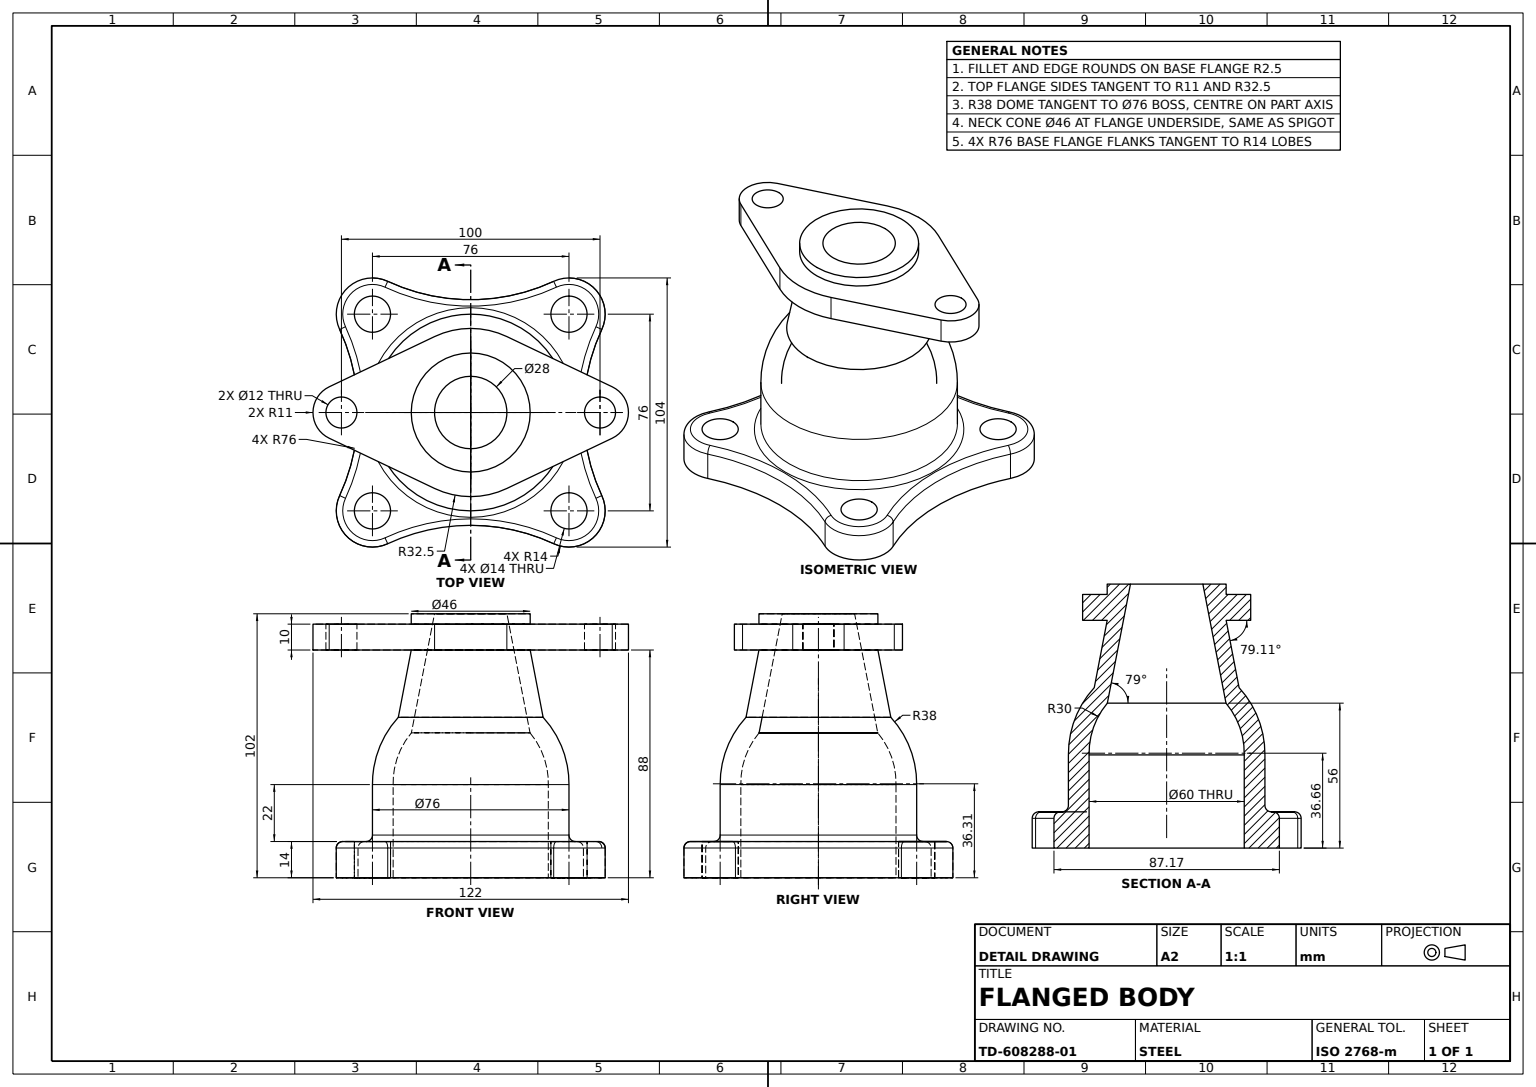
solid
v1 (0,0,-30)
v2 (0,36,-30)
e1 v1 v2 LINE
v3 (0,0,30)
e2 v3 v1 CIRCLE(AX(P(0,0,0),D(0,1,0),D(0,0,1)),30)
v4 (0,36,30)
e3 v3 v4 LINE
e4 v4 v2 CIRCLE(AX(P(0,36,0),D(0,1,0),D(0,0,1)),30)
face CYL(AX(P(0,0,0),D(0,1,0),D(0,0,1)),30) rev [-e1 -e2 e3 e4]
v5 (-38,0,45)
v6 (-38,14,45)
e5 v5 v6 LINE
v7 (-38,14,31)
e6 v6 v7 CIRCLE(AX(P(-38,14,38),D(0,1,0),D(0,0,1)),7)
v8 (-38,0,31)
e7 v8 v7 LINE
e8 v5 v8 CIRCLE(AX(P(-38,0,38),D(0,1,0),D(0,0,1)),7)
face CYL(AX(P(-38,0,38),D(0,1,0),D(0,0,1)),7) rev [e5 e6 -e7 -e8]
v9 (38,0,31)
v10 (38,14,31)
e9 v9 v10 LINE
v11 (38,0,45)
e10 v11 v9 CIRCLE(AX(P(38,0,38),D(0,1,0),D(0,0,1)),7)
v12 (38,14,45)
e11 v11 v12 LINE
e12 v12 v10 CIRCLE(AX(P(38,14,38),D(0,1,0),D(0,0,1)),7)
face CYL(AX(P(38,0,38),D(0,1,0),D(0,0,1)),7) rev [-e9 -e10 e11 e12]
v13 (0,11.5,43.584312)
v14 (0,14,41.084312)
e13 v13 v14 CIRCLE(AX(P(0,11.5,41.084312),D(-1,0,0),D(0,0,1)),2.5)
v15 (32.088889,11.5,50.690893)
e14 v15 v13 CIRCLE(AX(P(0,11.5,119.584312),D(0,1,0),D(0,0,-1)),76)
v16 (33.144444,14,48.424662)
e15 v16 v15 CIRCLE(AX(P(33.144444,11.5,48.424662),D(0.906492358,0,0.422222222),D(0.422222222,0,-0.906492358)),2.5)
e16 v14 v16 CIRCLE(AX(P(0,14,119.584312),D(0,-1,0),D(0,0,-1)),78.5)
face TORUS(AX(P(0,11.5,119.584312),D(0,-1,0),D(0,0,-1)),78.5,2.5) [-e13 -e14 -e15 -e16]
v17 (0,102,-14)
v18 (0,56,-22.941494)
e17 v17 v18 LINE
v19 (0,56,22.941494)
e18 v19 v18 CIRCLE(AX(P(0,56,0),D(0,1,0),D(0,0,1)),22.941494)
v20 (0,102,14)
e19 v20 v19 LINE
e20 v20 v17 CIRCLE(AX(P(0,102,0),D(0,1,0),D(0,0,1)),14)
face CONE(AX(P(0,56,0),D(0,-1,0),D(0,0,-1)),22.94149422,0.191986218) rev [e17 -e18 -e19 e20]
v21 (-48.424662,14,33.144444)
v22 (-33.144444,14,48.424662)
e21 v21 v22 CIRCLE(AX(P(-38,14,38),D(0,1,0),D(0,0,-1)),11.5)
v23 (-50.690893,11.5,32.088889)
e22 v21 v23 CIRCLE(AX(P(-48.424662,11.5,33.144444),D(-0.422222222,0,0.906492358),D(0.906492358,0,0.422222222)),2.5)
v24 (-32.088889,11.5,50.690893)
e23 v24 v23 CIRCLE(AX(P(-38,11.5,38),D(0,-1,0),D(0,0,-1)),14)
e24 v22 v24 CIRCLE(AX(P(-33.144444,11.5,48.424662),D(0.906492358,0,-0.422222222),D(-0.422222222,0,-0.906492358)),2.5)
face TORUS(AX(P(-38,11.5,38),D(0,-1,0),D(0,0,-1)),11.5,2.5) [-e21 e22 -e23 -e24]
v25 (54.73,98,-9.931118)
v26 (54.73,88,-9.931118)
e25 v25 v26 LINE
v27 (13.975,88,-29.341939)
e26 v26 v27 LINE
v28 (13.975,98,-29.341939)
e27 v28 v27 LINE
e28 v25 v28 LINE
face PLANE(AX(P(13.975,98,-29.341939),D(-0.43,0,0.902828887),D(0.902828887,0,0.43))) rev [e25 e26 -e27 -e28]
v29 (-38,11.5,-52)
v30 (-32.088889,11.5,-50.690893)
e29 v29 v30 CIRCLE(AX(P(-38,11.5,-38),D(0,-1,0),D(0,0,-1)),14)
v31 (-32.088889,0,-50.690893)
e30 v30 v31 LINE
v32 (-38,0,-52)
e31 v31 v32 CIRCLE(AX(P(-38,0,-38),D(0,1,0),D(0,0,1)),14)
e32 v29 v32 LINE
face CYL(AX(P(-38,14,-38),D(0,-1,0),D(0,0,-1)),14) [e29 e30 e31 -e32]
v33 (0,36,38)
v34 (0,16.5,38)
e33 v33 v34 LINE
v35 (0,16.5,-38)
e34 v34 v35 CIRCLE(AX(P(0,16.5,0),D(0,1,0),D(0,0,-1)),38)
v36 (0,36,-38)
e35 v36 v35 LINE
e36 v33 v36 CIRCLE(AX(P(0,36,0),D(0,1,0),D(0,0,1)),38)
face CYL(AX(P(0,36,0),D(0,-1,0),D(0,0,-1)),38) [e33 e34 -e35 -e36]
e37 v9 v11 CIRCLE(AX(P(38,0,38),D(0,1,0),D(0,0,1)),7)
e38 v10 v12 CIRCLE(AX(P(38,14,38),D(0,1,0),D(0,0,1)),7)
face CYL(AX(P(38,0,38),D(0,1,0),D(0,0,1)),7) rev [-e11 -e37 e9 e38]
e39 v17 v20 CIRCLE(AX(P(0,102,0),D(0,1,0),D(0,0,1)),14)
e40 v18 v19 CIRCLE(AX(P(0,56,0),D(0,1,0),D(0,0,1)),22.941494)
face CONE(AX(P(0,56,0),D(0,-1,0),D(0,0,-1)),22.94149422,0.191986218) rev [-e17 e39 e19 -e40]
v37 (50.690893,11.5,32.088889)
e41 v37 v15 CIRCLE(AX(P(38,11.5,38),D(0,-1,0),D(0,0,-1)),14)
v38 (48.424662,14,33.144444)
e42 v37 v38 CIRCLE(AX(P(48.424662,11.5,33.144444),D(0.422222222,0,0.906492358),D(0.906492358,0,-0.422222222)),2.5)
e43 v16 v38 CIRCLE(AX(P(38,14,38),D(0,1,0),D(0,0,-1)),11.5)
face TORUS(AX(P(38,11.5,38),D(0,-1,0),D(0,0,-1)),11.5,2.5) [e15 -e41 e42 -e43]
v39 (54.73,98,9.931118)
v40 (54.73,88,9.931118)
e44 v39 v40 LINE
v41 (13.975,98,29.341939)
e45 v41 v39 LINE
v42 (13.975,88,29.341939)
e46 v41 v42 LINE
e47 v42 v40 LINE
face PLANE(AX(P(13.975,98,29.341939),D(-0.43,0,-0.902828887),D(-0.902828887,0,0.43))) rev [-e44 -e45 e46 e47]
v43 (32.088889,0,50.690893)
e48 v15 v43 LINE
v44 (50.690893,0,32.088889)
e49 v43 v44 CIRCLE(AX(P(38,0,38),D(0,1,0),D(0,0,1)),14)
e50 v37 v44 LINE
face CYL(AX(P(38,14,38),D(0,-1,0),D(0,0,-1)),14) [e41 e48 e49 -e50]
v45 (-54.73,98,9.931118)
v46 (-13.975,98,29.341939)
e51 v45 v46 LINE
v47 (-54.73,88,9.931118)
e52 v45 v47 LINE
v48 (-13.975,88,29.341939)
e53 v47 v48 LINE
e54 v46 v48 LINE
face PLANE(AX(P(-54.73,98,9.931118),D(0.43,0,-0.902828887),D(-0.902828887,0,-0.43))) rev [-e51 e52 e53 -e54]
v49 (-50,98,-6)
v50 (-50,98,6)
e55 v49 v50 CIRCLE(AX(P(-50,98,0),D(0,1,0),D(0,0,1)),6)
e56 v50 v49 CIRCLE(AX(P(-50,98,0),D(0,1,0),D(0,0,1)),6)
v51 (-13.975,98,-29.341939)
v52 (-54.73,98,-9.931118)
e57 v51 v52 LINE
e58 v52 v45 CIRCLE(AX(P(-50,98,0),D(0,1,0),D(0,0,1)),11)
e59 v46 v41 CIRCLE(AX(P(0,98,0),D(0,1,0),D(0,0,1)),32.5)
e60 v39 v25 CIRCLE(AX(P(50,98,0),D(0,1,0),D(0,0,1)),11)
v53 (0,98,-32.5)
e61 v28 v53 CIRCLE(AX(P(0,98,0),D(0,1,0),D(0,0,1)),32.5)
e62 v53 v51 CIRCLE(AX(P(0,98,0),D(0,1,0),D(0,0,1)),32.5)
v54 (0,98,-23)
v55 (0,98,23)
e63 v54 v55 CIRCLE(AX(P(0,98,0),D(0,1,0),D(0,0,1)),23)
e64 v55 v54 CIRCLE(AX(P(0,98,0),D(0,1,0),D(0,0,1)),23)
v56 (50,98,6)
v57 (50,98,-6)
e65 v56 v57 CIRCLE(AX(P(50,98,0),D(0,1,0),D(0,0,1)),6)
e66 v57 v56 CIRCLE(AX(P(50,98,0),D(0,1,0),D(0,0,1)),6)
face PLANE(AX(P(-50,98,0),D(0,1,0),D(0,0,1))) [-e55 -e56] [e57 e58 e51 e59 e45 e60 e28 e61 e62] [-e63 -e64] [-e65 -e66]
v58 (-38,14,-49.5)
e67 v58 v29 CIRCLE(AX(P(-38,11.5,-49.5),D(-1,0,0),D(0,0,1)),2.5)
v59 (-33.144444,14,-48.424662)
e68 v59 v58 CIRCLE(AX(P(-38,14,-38),D(0,1,0),D(0,0,-1)),11.5)
e69 v30 v59 CIRCLE(AX(P(-33.144444,11.5,-48.424662),D(0.906492358,0,0.422222222),D(0.422222222,0,-0.906492358)),2.5)
face TORUS(AX(P(-38,11.5,-38),D(0,-1,0),D(0,0,-1)),11.5,2.5) [-e29 -e67 -e68 -e69]
v60 (50.690893,11.5,-32.088889)
e70 v60 v37 CIRCLE(AX(P(119.584312,11.5,0),D(0,1,0),D(0,0,-1)),76)
v61 (48.424662,14,-33.144444)
e71 v60 v61 CIRCLE(AX(P(48.424662,11.5,-33.144444),D(-0.422222222,0,0.906492358),D(0.906492358,0,0.422222222)),2.5)
e72 v38 v61 CIRCLE(AX(P(119.584312,14,0),D(0,-1,0),D(0,0,-1)),78.5)
face TORUS(AX(P(119.584312,11.5,0),D(0,-1,0),D(0,0,-1)),78.5,2.5) [-e70 e71 -e72 -e42]
v62 (0,102,-23)
v63 (0,102,23)
e73 v62 v63 CIRCLE(AX(P(0,102,0),D(0,1,0),D(0,0,1)),23)
e74 v63 v62 CIRCLE(AX(P(0,102,0),D(0,1,0),D(0,0,1)),23)
face PLANE(AX(P(0,102,0),D(0,1,0),D(0,0,1))) [-e39 -e20] [e73 e74]
v64 (38,0,-52)
v65 (32.088889,0,-50.690893)
e75 v64 v65 CIRCLE(AX(P(38,0,-38),D(0,1,0),D(0,0,1)),14)
v66 (32.088889,11.5,-50.690893)
e76 v66 v65 LINE
v67 (38,11.5,-52)
e77 v66 v67 CIRCLE(AX(P(38,11.5,-38),D(0,-1,0),D(0,0,-1)),14)
e78 v67 v64 LINE
face CYL(AX(P(38,14,-38),D(0,-1,0),D(0,0,-1)),14) [e75 -e76 e77 e78]
v68 (0,14,40.5)
e79 v68 v34 CIRCLE(AX(P(0,16.5,40.5),D(1,0,0),D(0,0,-1)),2.5)
e80 v35 v34 CIRCLE(AX(P(0,16.5,0),D(0,1,0),D(0,0,-1)),38)
v69 (0,14,-40.5)
e81 v69 v35 CIRCLE(AX(P(0,16.5,-40.5),D(-1,0,0),D(0,0,1)),2.5)
e82 v68 v69 CIRCLE(AX(P(0,14,0),D(0,-1,0),D(0,0,-1)),40.5)
face TORUS(AX(P(0,16.5,0),D(0,-1,0),D(0,0,-1)),40.5,2.5) rev [e79 -e80 -e81 -e82]
e83 v69 v68 CIRCLE(AX(P(0,14,0),D(0,-1,0),D(0,0,-1)),40.5)
face TORUS(AX(P(0,16.5,0),D(0,-1,0),D(0,0,-1)),40.5,2.5) rev [-e79 -e83 e81 -e34]
v70 (-38,0,-31)
v71 (-38,14,-31)
e84 v70 v71 LINE
v72 (-38,0,-45)
e85 v72 v70 CIRCLE(AX(P(-38,0,-38),D(0,1,0),D(0,0,1)),7)
v73 (-38,14,-45)
e86 v72 v73 LINE
e87 v73 v71 CIRCLE(AX(P(-38,14,-38),D(0,1,0),D(0,0,1)),7)
face CYL(AX(P(-38,0,-38),D(0,1,0),D(0,0,1)),7) rev [-e84 -e85 e86 e87]
v74 (0,88,23)
v75 (0,62,28)
e88 v74 v75 LINE
v76 (0,88,-23)
e89 v76 v74 CIRCLE(AX(P(0,88,0),D(0,1,0),D(0,0,1)),23)
v77 (0,62,-28)
e90 v76 v77 LINE
e91 v77 v75 CIRCLE(AX(P(0,62,0),D(0,1,0),D(0,0,1)),28)
face CONE(AX(P(0,88,0),D(0,-1,0),D(0,0,-1)),23,0.189988288) [-e88 -e89 e90 e91]
e92 v63 v55 LINE
e93 v62 v54 LINE
face CYL(AX(P(0,102,0),D(0,-1,0),D(0,0,-1)),23) [e63 -e92 -e73 e93]
e94 v13 v24 CIRCLE(AX(P(0,11.5,119.584312),D(0,1,0),D(0,0,-1)),76)
e95 v22 v14 CIRCLE(AX(P(0,14,119.584312),D(0,-1,0),D(0,0,-1)),78.5)
face TORUS(AX(P(0,11.5,119.584312),D(0,-1,0),D(0,0,-1)),78.5,2.5) [-e94 e13 -e95 e24]
v78 (-50.690893,11.5,-32.088889)
e96 v78 v29 CIRCLE(AX(P(-38,11.5,-38),D(0,-1,0),D(0,0,-1)),14)
v79 (-48.424662,14,-33.144444)
e97 v79 v78 CIRCLE(AX(P(-48.424662,11.5,-33.144444),D(0.422222222,0,0.906492358),D(0.906492358,0,-0.422222222)),2.5)
e98 v58 v79 CIRCLE(AX(P(-38,14,-38),D(0,1,0),D(0,0,-1)),11.5)
face TORUS(AX(P(-38,11.5,-38),D(0,-1,0),D(0,0,-1)),11.5,2.5) [e67 -e96 -e97 -e98]
e99 v7 v6 CIRCLE(AX(P(-38,14,38),D(0,1,0),D(0,0,1)),7)
e100 v8 v5 CIRCLE(AX(P(-38,0,38),D(0,1,0),D(0,0,1)),7)
face CYL(AX(P(-38,0,38),D(0,1,0),D(0,0,1)),7) rev [e99 -e5 -e100 e7]
e101 v67 v60 CIRCLE(AX(P(38,11.5,-38),D(0,-1,0),D(0,0,-1)),14)
v80 (38,14,-49.5)
e102 v80 v67 CIRCLE(AX(P(38,11.5,-49.5),D(-1,0,0),D(0,0,1)),2.5)
e103 v61 v80 CIRCLE(AX(P(38,14,-38),D(0,1,0),D(0,0,-1)),11.5)
face TORUS(AX(P(38,11.5,-38),D(0,-1,0),D(0,0,-1)),11.5,2.5) [-e101 -e102 -e103 -e71]
e104 v1 v3 CIRCLE(AX(P(0,0,0),D(0,1,0),D(0,0,1)),30)
e105 v2 v4 CIRCLE(AX(P(0,36,0),D(0,1,0),D(0,0,1)),30)
face CYL(AX(P(0,0,0),D(0,1,0),D(0,0,1)),30) rev [-e3 -e104 e1 e105]
e106 v40 v26 CIRCLE(AX(P(50,88,0),D(0,1,0),D(0,0,1)),11)
face CYL(AX(P(50,98,0),D(0,-1,0),D(0,0,-1)),11) [e106 -e25 -e60 e44]
v81 (0,88,-32.5)
e107 v27 v81 CIRCLE(AX(P(0,88,0),D(0,1,0),D(0,0,1)),32.5)
e108 v53 v81 LINE
face CYL(AX(P(0,98,0),D(0,-1,0),D(0,0,-1)),32.5) [-e61 e27 e107 -e108]
v82 (-50.690893,0,-32.088889)
e109 v78 v82 LINE
e110 v32 v82 CIRCLE(AX(P(-38,0,-38),D(0,1,0),D(0,0,1)),14)
face CYL(AX(P(-38,14,-38),D(0,-1,0),D(0,0,-1)),14) [-e109 e96 e32 e110]
v83 (-50,88,-6)
e111 v83 v49 LINE
v84 (-50,88,6)
e112 v84 v50 LINE
e113 v84 v83 CIRCLE(AX(P(-50,88,0),D(0,-1,0),D(0,0,1)),6)
face CYL(AX(P(-50,-0.001,0),D(0,1,0),D(0,0,1)),6) rev [e111 e55 -e112 e113]
v85 (50.690893,0,-32.088889)
e114 v60 v85 LINE
e115 v85 v64 CIRCLE(AX(P(38,0,-38),D(0,1,0),D(0,0,1)),14)
face CYL(AX(P(38,14,-38),D(0,-1,0),D(0,0,-1)),14) [-e78 e101 e114 e115]
e116 v30 v66 CIRCLE(AX(P(0,11.5,-119.584312),D(0,1,0),D(0,0,-1)),76)
e117 v65 v31 CIRCLE(AX(P(0,0,-119.584312),D(0,-1,0),D(0,0,1)),76)
face CYL(AX(P(0,14,-119.584312),D(0,-1,0),D(0,0,-1)),76) rev [-e30 e116 e76 e117]
e118 v44 v85 CIRCLE(AX(P(119.584312,0,0),D(0,-1,0),D(0,0,1)),76)
face CYL(AX(P(119.584312,14,0),D(0,-1,0),D(0,0,-1)),76) rev [e70 e50 e118 -e114]
v86 (-50.690893,0,32.088889)
e119 v82 v86 CIRCLE(AX(P(-119.584312,0,0),D(0,-1,0),D(0,0,-1)),76)
e120 v23 v86 LINE
e121 v23 v78 CIRCLE(AX(P(-119.584312,11.5,0),D(0,1,0),D(0,0,-1)),76)
face CYL(AX(P(-119.584312,14,0),D(0,-1,0),D(0,0,-1)),76) rev [e119 -e120 e121 e109]
v87 (33.144444,14,-48.424662)
e122 v66 v87 CIRCLE(AX(P(33.144444,11.5,-48.424662),D(0.906492358,0,-0.422222222),D(-0.422222222,0,-0.906492358)),2.5)
e123 v80 v87 CIRCLE(AX(P(38,14,-38),D(0,1,0),D(0,0,-1)),11.5)
face TORUS(AX(P(38,11.5,-38),D(0,-1,0),D(0,0,-1)),11.5,2.5) [e102 -e77 e122 -e123]
e124 v4 v19 CIRCLE(AX(P(0,36.660369,0.007269),D(-1,0,0),D(0,0,1)),30)
e125 v2 v18 CIRCLE(AX(P(0,36.660369,-0.007269),D(1,0,0),D(0,0,-1)),30)
face TORUS(AX(P(0,36.660369,0),D(0,1,0),D(0,0,1)),0.007269,30) rev [-e4 e124 e18 -e125]
v88 (0,0,43.584312)
e126 v13 v88 LINE
e127 v88 v43 CIRCLE(AX(P(0,0,119.584312),D(0,-1,0),D(0,0,-1)),76)
face CYL(AX(P(0,14,119.584312),D(0,-1,0),D(0,0,-1)),76) rev [e14 e126 e127 -e48]
e128 v83 v84 CIRCLE(AX(P(-50,88,0),D(0,-1,0),D(0,0,1)),6)
face CYL(AX(P(-50,-0.001,0),D(0,1,0),D(0,0,1)),6) rev [-e111 e128 e112 e56]
v89 (-32.088889,0,50.690893)
e129 v24 v89 LINE
e130 v86 v89 CIRCLE(AX(P(-38,0,38),D(0,1,0),D(0,0,1)),14)
face CYL(AX(P(-38,14,38),D(0,-1,0),D(0,0,-1)),14) [-e129 e23 e120 e130]
e131 v89 v88 CIRCLE(AX(P(0,0,119.584312),D(0,-1,0),D(0,0,-1)),76)
face CYL(AX(P(0,14,119.584312),D(0,-1,0),D(0,0,-1)),76) rev [-e126 e94 e129 e131]
v90 (-54.73,88,-9.931118)
e132 v90 v47 CIRCLE(AX(P(-50,88,0),D(0,1,0),D(0,0,1)),11)
e133 v52 v90 LINE
face CYL(AX(P(-50,98,0),D(0,-1,0),D(0,0,-1)),11) [e132 -e52 -e58 e133]
v91 (50,88,6)
e134 v91 v56 LINE
v92 (50,88,-6)
e135 v91 v92 CIRCLE(AX(P(50,88,0),D(0,-1,0),D(0,0,1)),6)
e136 v92 v57 LINE
face CYL(AX(P(50,-0.001,0),D(0,1,0),D(0,0,1)),6) rev [e66 -e134 e135 e136]
v93 (-13.975,88,-29.341939)
e137 v51 v93 LINE
e138 v93 v90 LINE
face PLANE(AX(P(-54.73,98,-9.931118),D(0.43,0,0.902828887),D(0.902828887,0,-0.43))) rev [-e57 e137 e138 -e133]
v94 (38,0,-31)
v95 (38,0,-45)
e139 v94 v95 CIRCLE(AX(P(38,0,-38),D(0,1,0),D(0,0,1)),7)
e140 v95 v94 CIRCLE(AX(P(38,0,-38),D(0,1,0),D(0,0,1)),7)
e141 v70 v72 CIRCLE(AX(P(-38,0,-38),D(0,1,0),D(0,0,1)),7)
face PLANE(AX(P(-78.792156,0,19),D(0,-1,0),D(0,0,-1))) [e10 e37] [e139 e140] [e141 e85] [e2 e104] [-e118 -e49 -e127 -e131 -e130 -e119 -e110 -e31 -e117 -e75 -e115] [e8 e100]
e142 v92 v91 CIRCLE(AX(P(50,88,0),D(0,-1,0),D(0,0,1)),6)
e143 v74 v76 CIRCLE(AX(P(0,88,0),D(0,1,0),D(0,0,1)),23)
e144 v48 v42 CIRCLE(AX(P(0,88,0),D(0,1,0),D(0,0,1)),32.5)
e145 v81 v93 CIRCLE(AX(P(0,88,0),D(0,1,0),D(0,0,1)),32.5)
face PLANE(AX(P(-50,88,0),D(0,1,0),D(0,0,1))) rev [-e135 -e142] [-e113 -e128] [e143 e89] [-e106 -e47 -e144 -e53 -e132 -e138 -e145 -e107 -e26]
face CYL(AX(P(0,98,0),D(0,-1,0),D(0,0,-1)),32.5) [e54 e144 -e46 -e59]
e146 v71 v73 CIRCLE(AX(P(-38,14,-38),D(0,1,0),D(0,0,1)),7)
face CYL(AX(P(-38,0,-38),D(0,1,0),D(0,0,1)),7) rev [-e86 -e141 e84 e146]
e147 v79 v21 CIRCLE(AX(P(-119.584312,14,0),D(0,-1,0),D(0,0,-1)),78.5)
face TORUS(AX(P(-119.584312,11.5,0),D(0,-1,0),D(0,0,-1)),78.5,2.5) [e97 -e121 -e22 -e147]
e148 v77 v36 CIRCLE(AX(P(0,36.308173,-0.00125),D(-1,0,0),D(0,0,1)),38)
e149 v75 v77 CIRCLE(AX(P(0,62,0),D(0,1,0),D(0,0,1)),28)
e150 v75 v33 CIRCLE(AX(P(0,36.308173,0.00125),D(1,0,0),D(0,0,-1)),38)
face TORUS(AX(P(0,36.308173,0),D(0,-1,0),D(0,0,-1)),0.00125,38) [-e148 -e149 e150 e36]
face CYL(AX(P(50,-0.001,0),D(0,1,0),D(0,0,1)),6) rev [-e136 e142 e134 e65]
e151 v36 v33 CIRCLE(AX(P(0,36,0),D(0,1,0),D(0,0,1)),38)
face TORUS(AX(P(0,36.308173,0),D(0,-1,0),D(0,0,-1)),0.00125,38) [e151 -e150 -e91 e148]
face CYL(AX(P(0,36,0),D(0,-1,0),D(0,0,-1)),38) [e80 -e33 -e151 e35]
face CYL(AX(P(0,102,0),D(0,-1,0),D(0,0,-1)),23) [-e93 -e74 e92 e64]
face TORUS(AX(P(0,36.660369,0),D(0,1,0),D(0,0,1)),0.007269,30) rev [-e105 e125 e40 -e124]
e152 v87 v59 CIRCLE(AX(P(0,14,-119.584312),D(0,-1,0),D(0,0,-1)),78.5)
face TORUS(AX(P(0,11.5,-119.584312),D(0,-1,0),D(0,0,-1)),78.5,2.5) [-e116 e69 -e152 -e122]
face CONE(AX(P(0,88,0),D(0,-1,0),D(0,0,-1)),23,0.189988288) [-e143 e88 e149 -e90]
v96 (38,14,-45)
e153 v95 v96 LINE
v97 (38,14,-31)
e154 v96 v97 CIRCLE(AX(P(38,14,-38),D(0,1,0),D(0,0,1)),7)
e155 v94 v97 LINE
face CYL(AX(P(38,0,-38),D(0,1,0),D(0,0,1)),7) rev [e153 e154 -e155 -e140]
e156 v97 v96 CIRCLE(AX(P(38,14,-38),D(0,1,0),D(0,0,1)),7)
face CYL(AX(P(38,0,-38),D(0,1,0),D(0,0,1)),7) rev [-e139 e155 e156 -e153]
face PLANE(AX(P(-78.792156,14,19),D(0,-1,0),D(0,0,-1))) rev [-e6 -e99] [-e146 -e87] [-e38 -e12] [e82 e83] [e103 e123 e152 e68 e98 e147 e21 e95 e16 e43 e72] [-e156 -e154]
face CYL(AX(P(0,98,0),D(0,-1,0),D(0,0,-1)),32.5) [-e62 e108 e145 -e137]
